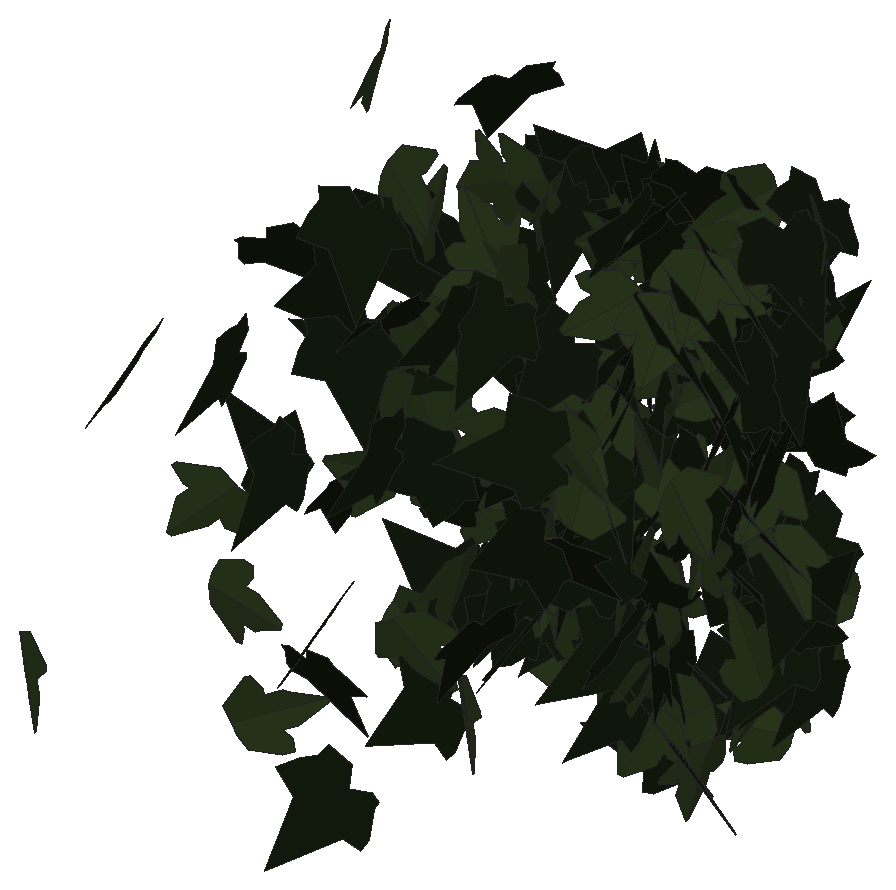
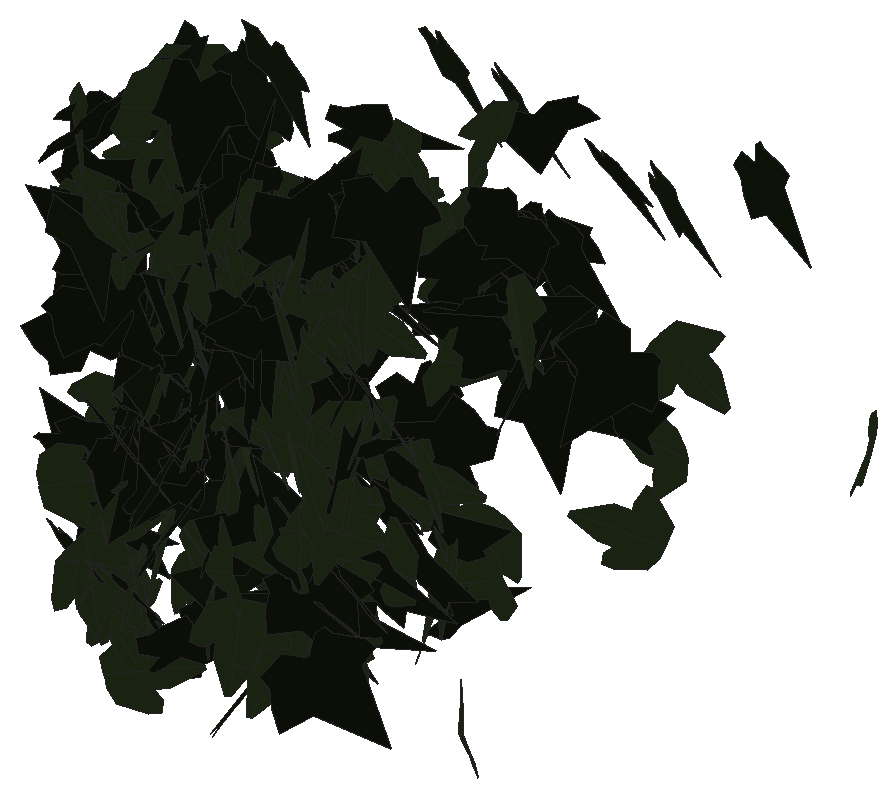
# SketchUp Ruby script. Lengths in inches.
U = 1.inch
M = Sketchup.active_model
def pt(a) = Geom::Point3d.new(a.map { |v| v * U })
def face(e, loops, mat)
  f = e.add_face(loops[0].map { |a| pt(a) })
  loops[1..].each { |l| e.add_face(l.map { |a| pt(a) }).erase! }
  f.material = f.back_material = mat if mat
  f
end
# faces: each face lists its corners as indices into pts; further lists are holes
def faces(e, pts, list, mat = nil) = list.each { |f| face(e, (f[0].is_a?(Array) ? f : [f]).map { |l| l.map { |i| pts[i] } }, mat) }
# xy, xz, yz: faces in a plane at the given z, y or x. An outline is a flat list of corners, or four numbers for a rectangle; further outlines are holes
def ring(l) = l.size == 4 ? [[l[0], l[1]], [l[2], l[1]], [l[2], l[3]], [l[0], l[3]]] : l.each_slice(2).to_a
def flat(e, list, mat, &to3) = list.each { |f| face(e, (f[0].is_a?(Array) ? f : [f]).map { |l| ring(l).map { |u, v| to3.(u, v) } }, mat) }
def xy(e, z, list, mat = nil) = flat(e, list, mat) { |x, y| [x, y, z] }
def xz(e, y, list, mat = nil) = flat(e, list, mat) { |x, z| [x, y, z] }
def yz(e, x, list, mat = nil) = flat(e, list, mat) { |y, z| [x, y, z] }
def lines(e, pts, list) = list.each { |a, b| e.add_line(pt(pts[a]), pt(pts[b])) }
# prism: a flat outline (further loops are holes) pulled along v
def prism(e, loops, v, mat = nil)
  f = face(e, loops, mat); d = Geom::Vector3d.new(v.map { |x| x * U })
  f.pushpull(f.normal.samedirection?(d) ? d.length : -d.length)
end
def box(e, o, s, mat = nil) = prism(e, [[o, [o[0] + s[0], o[1], o[2]], [o[0] + s[0], o[1] + s[1], o[2]], [o[0], o[1] + s[1], o[2]]]], [0, 0, s[2]], mat)
def at(x, y, z, deg = 0) = Geom::Transformation.translation(pt([x, y, z])) * Geom::Transformation.rotation(ORIGIN, Z_AXIS, deg.degrees)
def axes(o, x, y, z) = Geom::Transformation.new([*x, 0, *y, 0, *z, 0, *pt(o).to_a, 1])
def part(name) = M.definitions.add(name)
# library, detail: a bought-in or finely detailed component or shape, given as its bounding box
def library(name, o, s) = part(name).tap { |d| box(d.entities, o, s) }
def detail(e, o, s) = box(e.add_group.entities, o, s)
def put(e, d, t, mat = nil) = e.add_instance(d, t).tap { |i| i.material = mat if mat }
def group(e, t, mat = nil) = e.add_group.tap { |g| g.transformation = t; g.material = mat if mat }.entities
root = M.entities
M.materials.add("efeu1").color = [18, 25, 13]
M.materials.add("efeu2").color = [43, 57, 29]
c1 = part("ivyleaf_10")
p = [[0,0.5,-0.03],[-0.0625,2.02,-0.43],[-0.19,2.01,-0.46],[-0.54,1.05,-0.29],[-0.52,0.625,-0.18],[-0.83,0.76,-0.28],
  [-1.16,0.64,-0.33],[-1.15,0.33,-0.24],[-0.77,-0.39,0.02],[-0.3,-0.51,0.16],[0.04,-0.48,0.23],[-0.02,2.01,-0.4375],
  [-0.06,2.01,-0.43],[0.04,-0.49,0.23],[0.67,-0.49,0.14],[1.38,0.36,-0.2],[1.375,0.51,-0.24],[0.81,0.65,-0.19],
  [0.62,0.59,-0.15],[0.6,1.09,-0.28],[0.5,1.23,-0.31]]
faces(c1.entities,p,[[0,1,2,3,4,5,6,7,8,9,10],[11,12,0,13,14,15,16,17,18,19,20]],"efeu2")
c2 = part("ivyleaf_9")
p = [[1.54,2.16,1.25],[1.36,2.04,1.19],[-0.21,0.99,0.68],[-0.71,1.11,0.82],[-0.85,0.86,0.67],[-0.8,0.17,0.21],
  [-0.9,-0.01,0.1],[-0.67,-0.16,-0.02],[-0.08,-0.08,-0.05],[-0.03,-0.6,-0.4],[0.65,-0.88,-0.66],[0.83,-0.6,-0.49],
  [1.29,-0.42,-0.43],[1.8125,-0.07,-0.26],[1.21,0.44,0.15]]
faces(c2.entities,p,[[0,1,2,3,4,5,6,7,8,9,10,11,12,13,14]],"efeu1")
put(root,c1,axes([2.73,217.58,208.71],[-0.15867,0.36248,-0.19802],[0.08066,-0.17517,-0.40675],[-0.43478,-0.16478,-0.00319]))
put(root,c2,axes([6.96,218.19,208.07],[-0.37076,-0.24581,0.10884],[-0.09423,-0.0579,-0.4391],[0.27271,-0.35419,-0.00376]))
put(root,c2,axes([5.75,218.67,211.87],[-0.44387,0.03158,-0.14452],[0.14839,-0.02477,-0.42847],[-0.04085,-0.43314,0.01396]))
put(root,c2,axes([3.59,218.58,212.51],[-0.28724,0.3131,-0.14875],[0.09129,-0.1158,-0.42712],[-0.36038,-0.27889,0.01036]))
put(root,c2,axes([6.25,218.44,209.43],[0.45188,0.06138,-0.106],[-0.10897,-0.01446,-0.43981],[-0.06811,0.4304,0.00034]))
put(root,c2,axes([6.33,218.66,209.94],[-0.26733,0.33333,-0.135],[0.08358,-0.10422,-0.43179],[-0.37718,-0.25934,0]))
put(root,c2,axes([7.1875,218.77,212.44],[-0.40451,0.20996,-0.07245],[0.06388,-0.03695,-0.44655],[-0.23022,-0.37918,0.0034]))
put(root,c2,axes([4.32,219.47,212.4],[-0.38979,0.19792,-0.14631],[0.12589,-0.07987,-0.42787],[-0.23005,-0.37905,0.01377]))
put(root,c1,axes([4.02,219.62,210.38],[-0.27056,-0.16221,0.32913],[-0.27333,-0.19063,-0.30997],[0.26982,-0.35577,0.01603]))
put(root,c1,axes([4.02,219.67,209.05],[-0.04855,0.02095,-0.44945],[0.42722,-0.17404,-0.05156],[-0.18931,-0.39812,-0.00111]))
put(root,c1,axes([4.55,219.47,207.61],[-0.125,-0.13003,0.4146],[0.28141,0.30172,0.18102],[-0.35482,0.2851,-0.00249]))
put(root,c2,axes([8.55,219.85,211.22],[0.03,-0.00342,-0.45146],[-0.4178,-0.19757,-0.02413],[-0.21274,0.38753,-0.01629]))
put(root,c2,axes([8.31,220.27,212.11],[-0.33937,-0.0259,0.31167],[-0.3166,-0.07077,-0.32604],[0.07281,-0.42842,0.03502]))
put(root,c2,axes([7.13,220.04,213.51],[-0.34083,0.29797,0.03034],[-0.02499,0.01799,-0.45137],[-0.32238,-0.31641,0.00291]))
put(root,c2,axes([6.66,220.42,211.38],[-0.08783,-0.05144,-0.44119],[-0.27711,-0.33945,0.09396],[-0.36907,0.26711,0.03444]))
put(root,c2,axes([8.22,220.32,210.77],[0.42576,0.17988,0.03968],[0.024,0.04298,-0.44959],[-0.19714,0.39372,0.03096]))
put(root,c2,axes([7.07,220.59,209.23],[-0.10481,0.36156,-0.2304],[0.05325,-0.21611,-0.38926],[-0.45485,-0.10861,0.00752]))
put(root,c1,axes([5.34,221.03,210.5],[-0.13416,-0.12467,-0.41372],[-0.26449,-0.3141,0.18191],[-0.36436,0.27391,0.02029]))
put(root,c2,axes([4.94,220.84,212.23],[-0.24041,-0.26514,-0.27393],[0.19156,0.19491,-0.35993],[0.35528,-0.2845,0.0087]))
put(root,c1,axes([7.31,220.84,211.87],[-0.32138,-0.27676,0.16136],[-0.11903,-0.10931,-0.42262],[0.32133,-0.3173,0.00484]))
put(root,c2,axes([3.97,220.76,210.11],[-0.02619,0.0602,0.44734],[-0.33302,0.30101,-0.06189],[-0.33034,-0.30821,0.02693]))
put(root,c2,axes([4.92,221.05,213.8125],[-0.16141,-0.39266,-0.11725],[0.03154,0.10947,-0.43679],[0.44007,-0.15186,-0.0117]))
put(root,c2,axes([4.86,220.97,210.28],[-0.01074,0.42298,-0.10511],[0.00344,-0.10102,-0.44002],[-0.46966,-0.01041,-0.00082]))
put(root,c2,axes([7.23,221,208.86],[-0.17724,0.402,0.02736],[-0.01131,0.02414,-0.45157],[-0.43494,-0.16444,0.00059]))
put(root,c1,axes([5.03,221.45,211.14],[0.20527,-0.23841,-0.32267],[0.22666,-0.22899,0.31671],[-0.35665,-0.28275,0.01557]))
put(root,c2,axes([5.16,221.13,212.4],[0.02852,0.42991,-0.06331],[-0.00664,-0.06061,-0.44794],[-0.46889,0.02701,0.00249]))
put(root,c2,axes([4.46,221.3125,212.47],[-0.01682,-0.01655,-0.45178],[-0.44219,-0.14552,0.02103],[-0.15778,0.4096,-0.01078]))
put(root,c1,axes([5.72,221.28,211.39],[-0.40686,-0.19023,-0.10966],[0.10666,0.03827,-0.43878],[0.20928,-0.38932,0.01045]))
put(root,c2,axes([5.62,221.76,207.26],[-0.2,-0.23711,0.32675],[-0.17475,-0.27066,-0.31163],[0.38752,-0.24442,0.02811]))
put(root,c1,axes([5.37,221.34,208.27],[-0.39532,-0.06836,-0.23387],[0.23827,0.04356,-0.38726],[0.08751,-0.42738,-0.00206]))
put(root,c1,axes([7.46,221.61,211.51],[-0.32352,0.10328,-0.30996],[0.29911,-0.11059,-0.32935],[-0.16304,-0.40783,0.01081]))
put(root,c1,axes([7.72,221.59,210.59],[0.46214,-0.05606,-0.05679],[0.05977,0.0022,0.44872],[-0.05975,-0.43137,0.00966]))
put(root,c2,axes([4.39,221.53,211.25],[0.30059,-0.20136,-0.27754],[-0.22392,0.16843,-0.35706],[0.28322,0.34686,0.01227]))
put(root,c2,axes([4.78,221.81,211.35],[-0.06892,0.00497,0.44748],[-0.46291,-0.03903,-0.06565],[0.04091,-0.43322,0.01104]))
put(root,c1,axes([5.21,221.94,211.86],[-0.14857,-0.27352,-0.32137],[-0.14855,-0.27671,0.31841],[-0.4202,0.19453,0.00106]))
put(root,c2,axes([7.875,221.61,209.53],[-0.21522,-0.13257,0.37776],[0.35577,0.15577,0.24708],[-0.21867,0.38391,0.03019]))
put(root,c2,axes([8.3,221.625,209.02],[-0.21571,0.37921,0.07739],[-0.05674,0.05634,-0.44525],[-0.41348,-0.20556,0.02072]))
put(root,c2,axes([6.3,221.96,212.6],[-0.40417,-0.20212,-0.09489],[0.0923,0.03369,-0.4422],[0.221,-0.38371,0.01116]))
put(root,c2,axes([8.18,221.96,208.79],[-0.45609,-0.05005,0.09521],[-0.09445,-0.03839,-0.44136],[0.06146,-0.4304,0.02829]))
put(root,c1,axes([5.78,221.9,207.33],[-0.17309,0.33324,-0.23828],[0.10599,-0.20704,-0.38456],[-0.4237,-0.18792,0.00114]))
put(root,c1,axes([4.85,221.88,208.03],[0.20753,-0.00443,0.40584],[0.42146,-0.00133,-0.19986],[0.0034,0.43498,0.00353]))
put(root,c1,axes([4.98,221.66,214.04],[-0.02185,0.39669,0.18444],[-0.02393,0.17637,-0.41291],[-0.46868,-0.0275,0.01248]))
put(root,c1,axes([5.67,221.91,208.97],[0.00814,-0.4349,0.00575],[0.0053,-0.00545,-0.45234],[0.4697,0.0076,0.00501]))
put(root,c2,axes([8.83,222.01,207.61],[0.28604,-0.28267,0.20585],[0.14743,-0.14334,-0.40285],[0.34228,0.29796,0.00149]))
put(root,c2,axes([7.72,222.17,210.36],[0.01817,-0.11951,0.43464],[0.09234,-0.40916,-0.12526],[0.46028,0.08681,0.00797]))
put(root,c1,axes([5.25,222.0625,211.51],[-0.08693,-0.04009,0.44263],[-0.37331,-0.24872,-0.09235],[0.27165,-0.35462,0.01474]))
put(root,c2,axes([8.24,222.02,208.12],[-0.45363,0.11104,-0.02262],[0.02217,-0.00742,-0.45183],[-0.12017,-0.42052,0.002]))
put(root,c1,axes([8.42,222.02,208.55],[0.00055,-0.43491,-0.00893],[0.00828,0.00859,-0.45224],[0.46973,0.00036,0.00798]))
put(root,c1,axes([9.03,221.84,211.1],[0.02284,0.40234,0.17058],[-0.01121,0.16463,-0.41861],[-0.46911,0.01566,0.0183]))
put(root,c1,axes([7.8,222.34,209.15],[-0.02027,0.02999,0.4509],[0.31621,-0.31983,0.03619],[0.34686,0.29332,-0.00664]))
put(root,c2,axes([5.58,222.0625,208.5],[-0.38585,-0.12278,-0.22429],[-0.21576,-0.08198,0.39272],[-0.15901,0.40918,0.01137]))
put(root,c2,axes([5.09,222.28,211.69],[-0.24892,-0.36312,-0.06782],[0.03951,0.05401,-0.44728],[0.39647,-0.23336,0.002]))
put(root,c1,axes([5.53,221.93,212.47],[-0.18997,-0.13033,-0.39093],[0.36266,0.17178,-0.22536],[0.23043,-0.3778,0.03239]))
put(root,c2,axes([8.28,222.37,208.6875],[0.09428,-0.06677,-0.43772],[0.40282,-0.19583,0.11277],[-0.22261,-0.38264,0.01867]))
put(root,c2,axes([4.7,221.89,211.3125],[0.09703,0.01266,0.44245],[0.42465,0.164,-0.09143],[-0.17599,0.4027,0.02333]))
put(root,c2,axes([8.28,222.09,207.96],[0.42924,-0.17398,-0.03272],[-0.0311,0.01267,-0.45122],[0.1884,0.39849,0.00006]))
put(root,c1,axes([5.125,222.43,211.12],[0.11355,0.21049,-0.38051],[-0.17095,-0.32988,-0.24467],[-0.4226,0.19,-0.00327]))
put(root,c1,axes([5.4,222.07,208.21],[-0.33025,0.23477,0.20956],[-0.17518,0.1196,-0.40092],[-0.28454,-0.34612,0.0036]))
put(root,c1,axes([8.29,222.22,207.67],[0.41205,0.11537,-0.18118],[-0.21502,0.09066,-0.39103],[-0.06848,0.40951,0.13761]))
put(root,c2,axes([6.26,222.38,208.9375],[-0.44078,-0.0077,-0.15634],[0.16195,0.01692,-0.4243],[0.01412,-0.4346,-0.01375]))
put(root,c2,axes([5.08,222.16,209.63],[0.16626,-0.0137,0.42288],[0.43939,0.00756,-0.15993],[-0.0024,0.43472,0.01611]))
put(root,c2,axes([4.26,222.25,213.22],[-0.04802,-0.08712,-0.44082],[0.30439,0.31749,-0.09861],[0.35462,-0.28431,0.02496]))
put(root,c2,axes([7.96,222.14,214.09],[-0.18931,0.37053,0.15145],[-0.09791,0.11778,-0.42517],[-0.41867,-0.19509,0.03095]))
put(root,c2,axes([5.01,222.66,212.34],[-0.15093,-0.07663,0.42094],[-0.37783,-0.20359,-0.16571],[0.2349,-0.3767,0.00393]))
put(root,c1,axes([8.86,222.43,213.8125],[0.41981,0.18346,-0.06956],[-0.06817,-0.02295,-0.44698],[-0.19957,0.39375,0.00636]))
put(root,c2,axes([6.82,222.57,212.02],[-0.44958,-0.11611,-0.05153],[0.05408,0.00487,-0.44936],[0.12516,-0.41919,0.00905]))
put(root,c1,axes([8.3,222.47,213.01],[0.37683,0.23278,-0.11992],[-0.09827,-0.07134,-0.43613],[-0.26278,0.36049,-0.00888]))
put(root,c1,axes([5.59,222.57,209.45],[-0.03394,0.02321,0.45057],[-0.40296,-0.22313,-0.01572],[0.23913,-0.37269,0.03747]))
put(root,c1,axes([4.98,222.14,213.12],[0.00824,0.1751,-0.41405],[-0.04241,0.39684,0.18073],[0.46781,0.03289,0.02367]))
put(root,c2,axes([8.0625,222.55,212.94],[0.35062,-0.28952,0.00227],[0.005,0.00191,-0.45237],[0.31265,0.32465,0.00469]))
put(root,c2,axes([8.59,222.61,213.46],[0.26624,-0.35694,0.03373],[0.05931,-0.00128,-0.44878],[0.38251,0.24864,0.04611]))
put(root,c2,axes([5.62,222.36,208.17],[-0.14648,0.1461,0.4021],[-0.28387,0.28355,-0.20733],[-0.34449,-0.29577,-0.00013]))
put(root,c2,axes([2.53,222.34,212.03],[0.37413,0.2613,0.03191],[0.02526,0.01994,-0.45127],[-0.28302,0.3472,0.0019]))
put(root,c1,axes([8.69,222.68,207.1875],[-0.04164,-0.43057,0.05037],[0.00165,-0.04876,-0.44955],[0.46795,-0.03814,0.00607]))
put(root,c1,axes([5.82,222.7,212.4375],[-0.41081,0.07051,0.20686],[0.21098,-0.03743,0.40233],[0.08621,0.42761,0.00111]))
put(root,c1,axes([7.97,222.97,208.34],[0.02186,-0.03141,0.45073],[0.23602,-0.37426,-0.03882],[0.40562,0.21947,-0.0017]))
put(root,c2,axes([6.0625,223.03,210.66],[0.13966,-0.24789,-0.34658],[0.21548,-0.26904,0.28865],[-0.39342,-0.23536,0.03507]))
put(root,c1,axes([7.25,222.71,211.29],[0.42749,-0.05627,-0.17827],[-0.1831,0.02532,-0.41579],[0.06663,0.4306,0.00115]))
put(root,c2,axes([5.75,222.84,209.85],[-0.25957,-0.17744,-0.32884],[0.34117,0.08371,-0.29858],[0.19219,-0.38824,0.08592]))
put(root,c2,axes([7.85,222.46,207.63],[-0.03862,0.09581,0.43972],[-0.16977,0.39251,-0.10633],[-0.43635,-0.16119,0.00245]))
put(root,c1,axes([5.7,222.64,213.79],[-0.2113,0.04115,0.40179],[-0.41748,0.02284,-0.20612],[-0.04215,-0.43245,0.02735]))
put(root,c1,axes([5.3,222.74,209.89],[0.35574,-0.26485,-0.10698],[-0.08666,0.06436,-0.43957],[0.29437,0.33902,-0.00012]))
put(root,c1,axes([6.06,222.78,209.94],[-0.3574,-0.00948,0.29346],[0.30475,0.0033,0.34429],[-0.0101,0.43488,0.00379]))
put(root,c1,axes([7.93,222.99,211.15],[0.09004,-0.27416,-0.34037],[0.10426,-0.31272,0.29802],[-0.44915,-0.12755,0.00095]))
put(root,c1,axes([5.46,222.76,212.69],[0.07828,0.41881,0.09627],[-0.0214,-0.0905,0.44202],[0.46274,-0.07503,0.00416]))
put(root,c2,axes([6,222.76,208.11],[-0.20613,-0.08134,-0.39763],[-0.38792,-0.13137,0.21555],[-0.16656,0.40663,-0.00991]))
put(root,c2,axes([8.71,222.89,213.73],[0.3271,-0.33014,0.18444],[0.12303,-0.1377,-0.46465],[0.35759,0.34936,-0.00885]))
put(root,c1,axes([6.43,222.45,210.85],[0.06492,0.09825,0.43625],[0.0775,0.41534,-0.11186],[-0.45879,0.08406,0.04284]))
put(root,c1,axes([5.51,222.78,208.29],[0.01091,-0.03478,0.45083],[0.46553,0.05828,-0.00559],[-0.06226,0.42967,0.03725]))
put(root,c1,axes([8.73,222.77,213.28],[0.29258,0.34032,-0.00437],[-0.00522,-0.00152,-0.45237],[-0.36753,0.27094,0.00295]))
put(root,c1,axes([6.22,222.82,208.88],[0.14701,0.4048,-0.08595],[-0.03473,-0.07637,-0.44412],[-0.44485,0.13974,0.00627]))
put(root,c1,axes([7.375,222.86,212.7],[0.30811,0.01612,-0.34111],[-0.35295,-0.02866,-0.29709],[-0.03477,0.43376,-0.00695]))
put(root,c2,axes([7.49,222.61,212.04],[-0.16307,0.39535,0.10465],[-0.05696,0.08747,-0.43975],[-0.43689,-0.15897,0.01827]))
put(root,c2,axes([7.8,222.48,213.85],[0.10156,0.36194,0.2311],[0.02308,0.22328,-0.38762],[-0.45811,0.09148,0.03171]))
put(root,c2,axes([7.34,222.93,211.36],[-0.33914,0.19206,-0.24106],[0.20588,-0.13235,-0.38264],[-0.25161,-0.36718,0.01183]))
put(root,c2,axes([7.4,223.11,210.98],[-0.23402,-0.37654,0.02301],[0.00951,-0.03056,-0.45119],[0.40725,-0.21566,0.02376]))
put(root,c1,axes([7.81,223.05,212.25],[-0.13241,0.18707,-0.38801],[0.23154,-0.3054,-0.23253],[-0.38674,-0.24689,-0.00637]))
put(root,c1,axes([7.91,222.68,210.87],[-0.13251,0.14077,-0.4086],[-0.30315,0.27521,0.19372],[0.33355,0.30605,0.01373]))
put(root,c1,axes([8.5,222.82,207.67],[0.26885,-0.13146,-0.34489],[-0.32252,0.14442,-0.29266],[0.21076,0.3887,-0.0079]))
put(root,c2,axes([6.2,222.93,210.13],[-0.13999,0.09425,0.42058],[0.30617,-0.28947,0.16466],[0.32768,0.31073,0.02583]))
put(root,c2,axes([8.05,223.15,206.83],[-0.10041,-0.02783,0.441],[-0.41606,-0.17768,-0.09998],[0.1937,-0.39608,0.01386]))
put(root,c2,axes([8.34,223.17,210.74],[0.08769,-0.38192,0.19942],[0.0501,-0.18615,-0.40603],[0.45882,0.09332,0.00622]))
put(root,c1,axes([7.54,223.09,209.43],[0.21272,-0.35129,0.17097],[0.08617,-0.14374,-0.41885],[0.40992,0.21251,-0.00068]))
put(root,c2,axes([6.42,223.18,209.09],[-0.058,0.05337,-0.44549],[0.38159,-0.24255,-0.0775],[-0.26783,-0.35713,-0.01394]))
put(root,c1,axes([9.24,222.95,208.39],[-0.1261,0.48257,0.03499],[-0.00536,-0.03755,0.49856],[0.48381,0.12536,0.01464]))
put(root,c2,axes([9.22,223.24,212.07],[0.05035,-0.42166,-0.10004],[0.0738,-0.08835,0.43723],[-0.46123,-0.06017,0.05904]))
put(root,c2,axes([7.81,222.7,209.91],[-0.18183,0.39471,-0.07414],[-0.03115,0.0652,0.44628],[0.43207,0.17081,0.00097]))
put(root,c2,axes([7.99,223.3,207.76],[-0.05507,-0.04154,0.4472],[-0.08235,-0.42532,-0.05214],[0.45923,-0.08125,0.04428]))
put(root,c2,axes([6.78,223.01,210.39],[0.02808,0.20225,-0.39962],[-0.35231,-0.24496,-0.15705],[-0.30952,0.29718,0.14251]))
put(root,c1,axes([6.63,222.85,211.46],[0.08511,0.38085,0.20266],[0.02188,0.19459,-0.40406],[-0.46151,0.07946,0.01822]))
put(root,c2,axes([8.73,223.18,211.59],[-0.25273,0.19325,-0.3241],[0.25601,-0.20233,-0.31561],[-0.30215,-0.33308,0.00367]))
put(root,c1,axes([5.875,223.07,213.68],[-0.22561,-0.03792,0.39485],[-0.40064,-0.08112,-0.2207],[0.09645,-0.42568,0.00689]))
put(root,c1,axes([6.22,223.28,210.15],[-0.18173,-0.23058,0.34138],[-0.17879,-0.28431,-0.29596],[0.39462,-0.235,0.02312]))
put(root,c2,axes([5.86,223.39,209.99],[-0.20879,-0.38459,0.0653],[0.04568,-0.09039,-0.44033],[0.41837,-0.18207,0.08066]))
put(root,c1,axes([7.93,222.98,210.15],[0.38475,0.16191,-0.1976],[0.18375,0.08479,0.40692],[0.19728,-0.39474,0.00636]))
put(root,c1,axes([6.6875,222.97,211.23],[-0.20323,-0.30672,-0.25419],[0.13843,0.20811,-0.37423],[0.40031,-0.22768,0.00037]))
put(root,c1,axes([5.84,223.11,211.76],[0.13267,0.01214,-0.4338],[-0.43977,0.09856,-0.12174],[0.09854,0.42351,0.04076]))
put(root,c1,axes([8.18,223.23,209.44],[-0.26409,0.03929,0.37192],[0.37875,-0.07046,0.25744],[0.08671,0.42745,0.00826]))
put(root,c2,axes([7.34,222.98,210.98],[0.07657,-0.00487,-0.44632],[-0.45957,0.05586,-0.07377],[0.06038,0.43137,0.00451]))
put(root,c2,axes([5.92,223.15,212.3],[-0.39428,0.16639,0.17484],[-0.16741,0.06523,-0.41722],[-0.19295,-0.39659,0.00473]))
put(root,c1,axes([5.82,223.31,208.89],[-0.34977,0.1034,0.28224],[0.261,-0.12947,0.35123],[0.17393,0.40221,0.04051]))
put(root,c2,axes([7.49,223.34,210.24],[-0.46836,0.01453,0.03198],[-0.03354,-0.00876,-0.45115],[-0.01498,-0.43467,0.01016]))
put(root,c2,axes([7.37,223.05,210.47],[-0.21002,0.38053,0.08454],[-0.04643,0.06931,-0.44438],[-0.41767,-0.19905,0.00689]))
put(root,c1,axes([6.9,223.31,210.09],[0.42269,-0.15232,0.11788],[0.11639,-0.03558,-0.43673],[0.16882,0.4059,0.00595]))
put(root,c2,axes([8.39,223.53,211.33],[0.11663,-0.3309,0.35623],[0.13476,-0.32999,-0.35064],[0.46716,0.1778,0.01222]))
put(root,c1,axes([8.31,222.98,213.52],[-0.14858,-0.24359,-0.41059],[0.24035,0.33338,-0.28476],[0.4125,-0.282,0.01803]))
put(root,c1,axes([7.1875,223.34,210.2],[0.31404,0.29683,-0.13383],[-0.08905,-0.09932,-0.43202],[-0.33787,0.30208,-0.01053]))
put(root,c1,axes([8.56,223.23,210.8125],[-0.07477,-0.41521,-0.11407],[0.02719,0.10698,-0.43772],[0.46301,-0.07333,0.00729]))
put(root,c2,axes([9.31,222.98,210.77],[0.05596,0.001,0.44918],[0.13236,0.41708,-0.01629],[-0.44728,0.12355,0.05137]))
put(root,c1,axes([5.95,223.36,213.52],[0.15591,-0.41023,0.00998],[0.00348,-0.00904,-0.45229],[0.44316,0.1444,0.00004]))
put(root,c2,axes([6.07,223.54,213.42],[-0.11022,-0.42156,0.03441],[-0.00514,-0.03289,-0.45108],[0.45666,-0.10212,0.00322]))
put(root,c2,axes([7.27,222.98,211.21],[0.035,0.02997,0.45006],[0.1619,0.40645,-0.04095],[-0.43963,0.15207,0.02075]))
put(root,c1,axes([6.1,223.42,208.25],[-0.28442,-0.17862,0.30846],[-0.25682,-0.17754,-0.33078],[0.27178,-0.35468,0.01024]))
put(root,c1,axes([5.8,223.28,210.26],[-0.00066,0.4349,-0.00962],[0.00198,-0.00925,-0.45229],[-0.4698,-0.00065,-0.00189]))
put(root,c1,axes([5.81,223.3,210.24],[0.08753,0.42738,0.00253],[0.00133,0.00225,-0.45239],[-0.46157,0.08105,-0.00082]))
put(root,c1,axes([8.14,223.49,209.76],[0.00013,0.37113,-0.23598],[-0.04522,-0.22584,-0.38419],[-0.46762,0.02195,0.03709]))
put(root,c1,axes([6.26,223.09,207.99],[-0.10688,0.17779,0.39986],[-0.19508,0.33942,-0.21158],[-0.4138,-0.20594,-0.00353]))
put(root,c1,axes([6.75,223.37,207.2],[-0.10499,-0.01856,0.44053],[-0.45714,-0.021,-0.10199],[0.0266,-0.4341,-0.01391]))
put(root,c2,axes([8.37,223.14,212.74],[0.3365,0.29124,0.08901],[0.06719,0.05877,-0.44356],[-0.32088,0.31773,0.00046]))
put(root,c2,axes([5.85,223.28,211.09],[-0.29248,0.27781,0.20461],[-0.14565,0.14328,-0.40347],[-0.33757,-0.30252,-0.0032]))
put(root,c1,axes([6.82,223.41,210.91],[-0.40732,-0.11964,0.18797],[-0.1873,-0.05102,-0.41148],[0.14042,-0.4151,-0.00361]))
put(root,c2,axes([7.05,223.53,208.36],[0.4396,0.05155,0.15032],[-0.15558,-0.0128,0.42666],[0.0571,-0.43174,0.0053]))
put(root,c1,axes([8.37,223.51,211.59],[0.19847,0.08935,-0.39938],[-0.41032,-0.07314,-0.20678],[-0.11384,0.4194,0.04903]))
put(root,c1,axes([5.63,223.38,210.49],[-0.23659,0.37313,-0.04664],[0.02179,-0.04016,-0.44998],[-0.40529,-0.21998,0.00303]))
put(root,c2,axes([5.95,223.64,207.84],[-0.36895,-0.10733,0.25686],[-0.2534,-0.07715,-0.3724],[0.14273,-0.41443,0.00281]))
put(root,c2,axes([8.33,223.45,210.1875],[0.42493,-0.19907,0.17264],[0.15325,-0.07979,-0.4692],[0.21436,0.45167,-0.00679]))
put(root,c1,axes([8.99,223.5,210.64],[0.44407,0.08533,-0.11803],[-0.12283,-0.01024,-0.43654],[-0.09181,0.42643,0.01313]))
put(root,c2,axes([7.68,223.41,213.54],[0.24158,0.17665,-0.34176],[-0.26756,-0.21615,-0.29622],[-0.30127,0.33361,-0.01097]))
put(root,c1,axes([7.54,223.68,211.5],[-0.21758,-0.23409,-0.31859],[-0.22804,-0.2222,0.32101],[-0.34838,0.29164,-0.01115]))
put(root,c2,axes([7.7,223.39,212.68],[-0.1107,-0.1602,-0.40687],[0.22783,0.32947,-0.19779],[0.39566,-0.23454,0.00006]))
put(root,c1,axes([6.71,223.71,210.13],[0.27008,-0.26999,0.32274],[0.22319,-0.23319,-0.38185],[0.35671,0.35033,-0.00544]))
put(root,c2,axes([6.92,223.33,210.06],[-0.04381,-0.12634,0.43084],[0.44021,0.12952,0.08259],[-0.15813,0.39558,0.11056]))
put(root,c1,axes([3.83,223.7,207.13],[0.17572,-0.10661,0.40465],[0.34876,-0.21705,-0.20229],[0.26116,0.36159,-0.00212]))
put(root,c2,axes([9.12,223.58,212.5625],[-0.23508,-0.17537,-0.34664],[0.33052,0.14201,-0.28557],[0.23707,-0.37189,0.05441]))
put(root,c2,axes([8.98,223.13,210.74],[-0.11884,0.12121,-0.4703],[-0.34552,0.31916,0.16956],[0.34131,0.3653,0.00791]))
put(root,c2,axes([8.07,223.58,209.8],[-0.01773,-0.01886,-0.45165],[0.45652,0.10066,-0.02117],[0.10948,-0.42277,0.01511]))
put(root,c2,axes([7.95,223.68,211.05],[0.2694,-0.03406,-0.36893],[0.3827,-0.02233,0.26137],[-0.04092,-0.43309,0.01554]))
put(root,c2,axes([9.19,223.83,209.23],[-0.13368,-0.39916,0.12556],[0.04541,-0.13724,-0.42706],[0.44808,-0.10518,0.08074]))
put(root,c2,axes([6.4,223.26,207.375],[-0.05096,0.41944,-0.10941],[-0.01288,0.10453,0.43897],[0.46685,0.04867,0.00017]))
put(root,c2,axes([7.84,223.66,209.34],[0.24057,0.22415,0.3109],[-0.21781,-0.22085,0.32851],[0.3397,-0.30035,-0.00954]))
put(root,c1,axes([9.08,223.625,209.73],[-0.42365,-0.05364,-0.18741],[0.20302,-0.11927,-0.38866],[-0.00359,-0.41488,0.13596]))
put(root,c1,axes([6.2,223.59,212.92],[-0.39303,0.12606,-0.21033],[0.20305,-0.07497,-0.40044],[-0.15815,-0.40953,0.00857]))
put(root,c2,axes([6.14,223.75,207.98],[-0.46539,-0.03862,-0.04698],[0.04935,-0.0039,-0.44988],[0.04104,-0.43326,0.00824]))
put(root,c2,axes([7.13,223.69,207.9],[0.27007,-0.28365,0.22362],[0.2309,-0.09039,-0.38261],[0.30734,0.31717,0.09095]))
put(root,c1,axes([5.81,223.43,207.28],[0.06843,0.0161,0.44726],[0.36152,0.27136,-0.06186],[-0.29212,0.3396,0.02822]))
put(root,c2,axes([5.77,223.75,213.6],[-0.3268,-0.182,-0.2642],[0.23475,0.13148,-0.36724],[0.24249,-0.37257,-0.00054]))
put(root,c2,axes([7.9,223.43,210.99],[-0.12715,-0.07611,0.42826],[0.38297,0.20942,0.14569],[-0.24058,0.3736,0.00558]))
put(root,c1,axes([8.5,223.96,213.99],[0.10574,0.12235,-0.47313],[-0.2779,-0.38313,-0.16119],[-0.40198,0.29705,-0.01302]))
put(root,c1,axes([5.98,223.68,207.5],[-0.39964,-0.11857,0.20337],[-0.20125,-0.05929,-0.40411],[0.14318,-0.41431,-0.00037]))
put(root,c1,axes([7.84,223.76,211.2],[0.29429,-0.33585,0.04855],[0.0318,-0.03622,-0.44979],[0.36482,0.27408,0.00004]))
put(root,c1,axes([8.42,223.66,210.17],[-0.17392,0.39467,-0.09023],[0.03583,-0.08016,-0.44331],[-0.43495,-0.16442,-0.00045]))
put(root,c2,axes([7.92,223.53,214.25],[0.33088,0.23056,-0.21366],[-0.18571,-0.11301,-0.39859],[-0.27702,0.35114,0.012]))
put(root,c2,axes([9.05,223.76,213.76],[-0.03275,-0.36226,-0.24845],[0.07353,0.23254,-0.37572],[0.46285,-0.06257,0.0421]))
put(root,c1,axes([6.23,223.84,210.21],[0.18402,-0.39529,0.06525],[0.02711,-0.0575,-0.44767],[0.43141,0.17223,0.0003]))
put(root,c1,axes([8.23,224.07,213.24],[-0.06998,0.07264,0.44093],[0.03692,-0.42653,0.08144],[0.46309,0.04498,0.06014]))
put(root,c1,axes([6.66,224.07,212.86],[-0.02872,-0.02806,-0.45061],[-0.23469,-0.37495,0.03912],[-0.40597,0.21875,0.00926]))
put(root,c2,axes([6.1,223.8,208.875],[-0.43591,0.15031,0.06342],[-0.05904,0.02793,-0.44787],[-0.16494,-0.40725,-0.00731]))
put(root,c2,axes([8.87,224.03,208.23],[-0.40231,-0.22274,-0.0303],[0.05367,-0.02669,-0.44858],[0.2366,-0.37269,0.05023]))
put(root,c2,axes([9.03,223.76,208.61],[-0.16095,-0.05844,0.46976],[0.46483,-0.11342,0.14515],[0.0896,0.48345,0.09084]))
put(root,c1,axes([8.9,223.78,212.36],[-0.45259,-0.09328,0.07286],[-0.07485,-0.01107,-0.44647],[0.10134,-0.42474,-0.00436]))
put(root,c2,axes([6.87,224.03,213.21],[-0.08194,0.16453,0.41129],[-0.14767,-0.38992,0.14142],[0.4384,-0.10059,0.12451]))
put(root,c1,axes([8.48,223.95,209.35],[0.39385,-0.11508,0.21564],[0.21678,-0.05272,-0.39759],[0.13637,0.41618,0.00926]))
put(root,c1,axes([7.56,223.95,210.12],[-0.11715,0.36675,-0.21554],[0.05249,-0.20169,-0.39764],[-0.45192,-0.1185,0.00969]))
put(root,c1,axes([6.93,224.15,212.8],[-0.06465,0.12166,0.42986],[-0.03937,-0.41723,0.12223],[0.46366,-0.01846,0.07031]))
put(root,c1,axes([6.79,223.82,213.11],[-0.43065,0.01538,0.18009],[-0.18743,-0.00965,-0.41472],[-0.01108,-0.43462,0.01558]))
put(root,c2,axes([6.1,223.8,208.85],[0.09094,0.4081,0.12983],[-0.04729,-0.11831,0.43296],[0.45848,-0.09316,0.0189]))
put(root,c1,axes([6.42,223.79,208.61],[0.40453,0.20436,-0.08801],[0.07947,0.04183,0.44375],[0.22528,-0.38172,0.00151]))
put(root,c1,axes([8.28,223.89,213.32],[0.42459,0.17321,0.07103],[0.06639,0.02986,-0.44678],[-0.18981,0.39791,0.00261]))
put(root,c1,axes([8.3,223.79,211.72],[0.20077,-0.22359,-0.33647],[-0.2291,0.24432,-0.30237],[0.35765,0.28202,-0.00481]))
put(root,c2,axes([7,223.82,211.75],[-0.06661,0.41321,-0.12601],[0.03337,-0.11783,-0.4343],[-0.46386,-0.06781,-0.01315]))
put(root,c2,axes([5.91,223.95,208.53],[0.1202,0.24546,-0.35511],[-0.14993,-0.31196,-0.28029],[-0.4287,0.17792,-0.00154]))
put(root,c1,axes([5.9375,224.14,209.29],[0.13557,0.16853,-0.39611],[-0.29261,-0.26908,-0.21669],[-0.34163,0.29735,0.02841]))
put(root,c1,axes([6.28,223.91,210.26],[-0.05174,-0.01055,0.44951],[0.44729,0.12371,0.05088],[-0.13403,0.41691,-0.00372]))
put(root,c1,axes([8.33,223.72,212.36],[0.20601,0.15518,-0.37318],[0.28206,0.24653,0.25526],[0.31419,-0.32306,0.01554]))
put(root,c2,axes([8.42,223.79,209.49],[-0.38276,0.2464,0.05606],[0.04476,-0.03481,0.44888],[0.2687,0.35679,0.00508]))
put(root,c2,axes([7.9,224.22,206.98],[-0.21834,-0.00507,0.40054],[-0.38612,-0.15934,-0.19737],[0.15474,-0.40474,0.07268]))
put(root,c2,axes([6,224.2,213.04],[0.18498,0.08686,0.45633],[-0.4235,-0.17027,0.20409],[0.19086,-0.46202,0.01058]))
put(root,c2,axes([9.08,224.125,211.34],[0.0018,0.17906,-0.41229],[-0.13855,-0.3786,-0.1784],[-0.4489,0.11758,0.05341]))
put(root,c2,axes([8.4375,223.86,210.375],[0.36433,-0.11247,-0.26057],[-0.24142,0.11812,-0.36815],[0.17233,0.40327,0.03515]))
put(root,c1,axes([6.31,224.03,211.98],[0.30037,-0.32565,-0.07937],[-0.04534,0.06448,-0.44527],[0.35837,0.2811,0.01019]))
put(root,c1,axes([7.58,223.76,207.6],[-0.12465,0.26551,-0.40493],[-0.17693,0.36424,0.2933],[0.45073,0.21641,0.00315]))
put(root,c1,axes([8.37,224.31,207.34],[0.04221,-0.31659,0.30758],[0.05259,-0.29186,-0.33161],[0.46494,0.06175,0.00959]))
put(root,c2,axes([8.08,223.91,208.95],[-0.15582,-0.20228,0.37134],[0.28775,0.24169,0.25437],[-0.33709,0.29982,0.04548]))
put(root,c2,axes([6.5,224.33,210.77],[0.02188,-0.03281,0.45062],[0.08041,-0.42708,-0.03726],[0.46235,0.07583,-0.01484]))
put(root,c2,axes([8.11,223.8,209.4],[0.3178,0.31042,0.0824],[0.05603,0.05999,-0.44482],[-0.34144,0.29877,0.0037]))
put(root,c2,axes([6.66,223.82,213.27],[0.07215,0.14703,-0.47242],[0.21865,0.41879,0.16373],[0.44383,-0.23021,-0.00387]))
put(root,c2,axes([8.375,224.01,212.5625],[-0.28822,0.18544,0.30073],[-0.25487,0.16712,-0.33797],[-0.2696,-0.35624,-0.00201]))
put(root,c1,axes([6.36,224.05,208.8],[0.27658,0.00758,0.36561],[-0.37975,0.0029,0.26633],[0.00229,-0.43492,0.00815]))
put(root,c2,axes([7.85,224.1,208.68],[0.2507,-0.33166,-0.16556],[-0.09499,0.13275,-0.421],[0.3858,0.2482,0.00393]))
put(root,c2,axes([9.36,224.21,207.99],[-0.44332,0.08059,-0.12407],[0.12774,-0.01676,-0.43501],[-0.08866,-0.42714,-0.00634]))
put(root,c1,axes([6.3125,224.04,207.58],[-0.26919,-0.31526,-0.17313],[0.14756,0.10314,-0.41589],[0.35563,-0.28143,0.04152]))
put(root,c2,axes([8.57,224.25,207.72],[-0.45568,0.03006,-0.10555],[0.1078,-0.0258,-0.43951],[-0.03804,-0.43319,0.01885]))
put(root,c2,axes([9.04,224.11,212.61],[0.08413,-0.00327,0.44507],[-0.40739,0.20495,0.07304],[-0.21834,-0.38368,0.03523]))
put(root,c2,axes([8.55,224.32,209.66],[-0.12215,0.17597,-0.39666],[0.21986,-0.32253,-0.21755],[-0.3968,-0.23288,0.00157]))
put(root,c1,axes([9.02,224.12,209.06],[0.20235,-0.37647,-0.11577],[-0.05441,0.09927,-0.43734],[0.42048,0.19401,-0.00087]))
put(root,c2,axes([9.24,224.37,209.52],[-0.41098,-0.16838,0.13181],[-0.11599,-0.07014,-0.43228],[0.19584,-0.39491,0.02058]))
put(root,c2,axes([9.03,224.21,210.72],[0.45661,0.07972,0.06677],[-0.07649,0.03086,0.44521],[0.0798,-0.42652,0.04469]))
put(root,c1,axes([9.18,224.19,212.67],[-0.27467,0.00411,0.367],[-0.36785,-0.11671,-0.25388],[0.09976,-0.41903,0.07431]))
put(root,c2,axes([6.61,224.05,211.77],[-0.01609,-0.24993,-0.36995],[0.02777,0.3548,-0.26038],[0.4687,-0.0296,0.00273]))
put(root,c1,axes([8.07,223.98,208.5],[-0.2515,0.31866,0.19021],[-0.10965,0.15229,-0.4104],[-0.38136,-0.25394,-0.00744]))
put(root,c2,axes([5.41,224.02,210.05],[-0.01371,-0.2413,0.37618],[0.08888,0.35399,0.2486],[-0.46111,0.07541,0.03673]))
put(root,c1,axes([8.37,224.14,207.81],[0.20407,-0.36806,-0.13974],[-0.0573,0.12377,-0.43018],[0.41927,0.19606,0.00923]))
put(root,c1,axes([6.7,224.4375,209.85],[0.0173,-0.03078,-0.45096],[0.23526,-0.37493,0.03605],[-0.40628,-0.21841,0.00167]))
put(root,c2,axes([8.96,223.99,211.99],[-0.02783,-0.09006,0.44179],[0.41398,0.19523,0.06723],[-0.22035,0.37815,0.07051]))
put(root,c2,axes([4.69,224.09,214.15],[0.05795,0.39862,-0.1723],[-0.05704,-0.15963,-0.41724],[-0.46271,0.0696,0.02986]))
put(root,c2,axes([5.59,224.37,207.77],[-0.00561,0.22712,-0.4454],[-0.03845,-0.44431,-0.22608],[-0.49849,0.03171,0.02245]))
put(root,c1,axes([9,224.29,207.87],[-0.17288,-0.46177,0.08296],[-0.03175,-0.0767,-0.49306],[0.46808,-0.17575,-0.0028]))
put(root,c1,axes([8.34,224.4,206.64],[0.06107,0.0866,0.43943],[-0.30444,-0.31512,0.1064],[0.35256,-0.2871,0.01576]))
put(root,c1,axes([6.73,224.34,213.39],[0.0489,0.36828,-0.23612],[-0.06022,-0.2214,-0.38508],[-0.46335,0.06764,0.02512]))
put(root,c1,axes([6.79,224.375,208.55],[0.16268,-0.09331,0.41317],[0.40383,-0.13808,-0.18117],[0.17655,0.40181,0.03368]))
put(root,c1,axes([9.34,224.36,208.85],[-0.09042,-0.01794,-0.44355],[-0.4406,-0.12456,0.08873],[-0.13569,0.4164,0.00743]))
put(root,c1,axes([6.0625,224.18,212.5625],[-0.30067,0.32507,-0.08091],[-0.05421,0.05944,0.44511],[0.35689,0.28288,-0.00056]))
put(root,c1,axes([6.99,224.28,212.875],[0.31017,0.3155,-0.08826],[-0.0619,-0.06259,-0.44371],[-0.34738,0.29286,0.00026]))
put(root,c1,axes([4.875,224.18,212.99],[-0.02166,-0.41568,-0.13168],[0.02083,0.12578,-0.43261],[0.46884,-0.02479,0.01314]))
put(root,c1,axes([8.51,224.57,208.59],[-0.01719,-0.01404,0.45186],[-0.00829,-0.4347,-0.0149],[0.46941,-0.00819,0.01629]))
put(root,c2,axes([8.11,224.47,208.9375],[0.17593,-0.40304,0.01637],[0.00939,0.02048,0.45181],[-0.43552,-0.16237,0.01635]))
put(root,c2,axes([6.53,224.37,207.08],[0.21228,-0.38763,-0.01907],[-0.01733,0.01242,-0.45191],[0.41875,0.19702,-0.00904]))
put(root,c1,axes([5.08,224.54,209.79],[0.07302,0.28114,-0.40697],[-0.13169,-0.38549,-0.28993],[-0.47679,0.14953,0.01775]))
put(root,c1,axes([7.52,224.46,212.96],[0.03759,0.31892,-0.30552],[-0.06611,-0.28815,-0.33288],[-0.4636,0.06695,0.02269]))
put(root,c2,axes([7.14,224.43,213.14],[-0.23634,0.10005,-0.37689],[0.35968,-0.14296,-0.2502],[-0.18839,-0.39847,-0.00487]))
put(root,c1,axes([8.55,224.25,207.71],[-0.4425,0.06437,-0.13643],[0.1358,-0.04365,-0.4307],[-0.0804,-0.42799,0.02341]))
put(root,c2,axes([8.95,224.5625,213.77],[-0.06971,-0.41221,0.12797],[0.00277,-0.12479,-0.43338],[0.46459,-0.06111,0.02178]))
put(root,c1,axes([9.33,224.06,213.64],[0.11879,-0.13579,-0.41429],[-0.19884,0.35473,-0.17862],[0.40874,0.21203,0.03351]))
put(root,c1,axes([8.31,224.1875,207.99],[-0.22805,0.37597,0.05962],[-0.03258,0.0488,-0.44845],[-0.40944,-0.21329,0.00248]))
put(root,c2,axes([8.84,224.21,209.79],[-0.32798,0.24911,0.19441],[-0.15593,0.11875,-0.4085],[-0.29804,-0.33626,-0.00023]))
put(root,c1,axes([4.94,224.33,213.14],[-0.0026,0.42473,-0.09769],[-0.02534,-0.09392,-0.44106],[-0.46911,0.00272,0.02437]))
put(root,c1,axes([5.35,224.41,209.72],[-0.34407,0.03362,0.36123],[0.35704,-0.05697,0.34537],[0.06438,0.49561,0.0152]))
put(root,c2,axes([9.14,224.14,212.38],[-0.09436,0.42222,0.05996],[-0.0349,0.05212,-0.44788],[-0.4589,-0.09078,0.02173]))
put(root,c1,axes([6.73,224.3125,207.91],[-0.4023,-0.22369,-0.02156],[0.01913,0.01077,-0.45189],[0.24187,-0.37292,-0.00012]))
put(root,c1,axes([2.55,224.34,213.64],[0.1571,-0.45522,-0.13452],[-0.05833,0.12211,-0.48134],[0.47108,0.16693,-0.01474]))
put(root,c1,axes([8.86,224.21,208.22],[-0.02295,0.41144,0.14519],[-0.04569,0.13715,-0.42707],[-0.46701,-0.03364,0.03464]))
